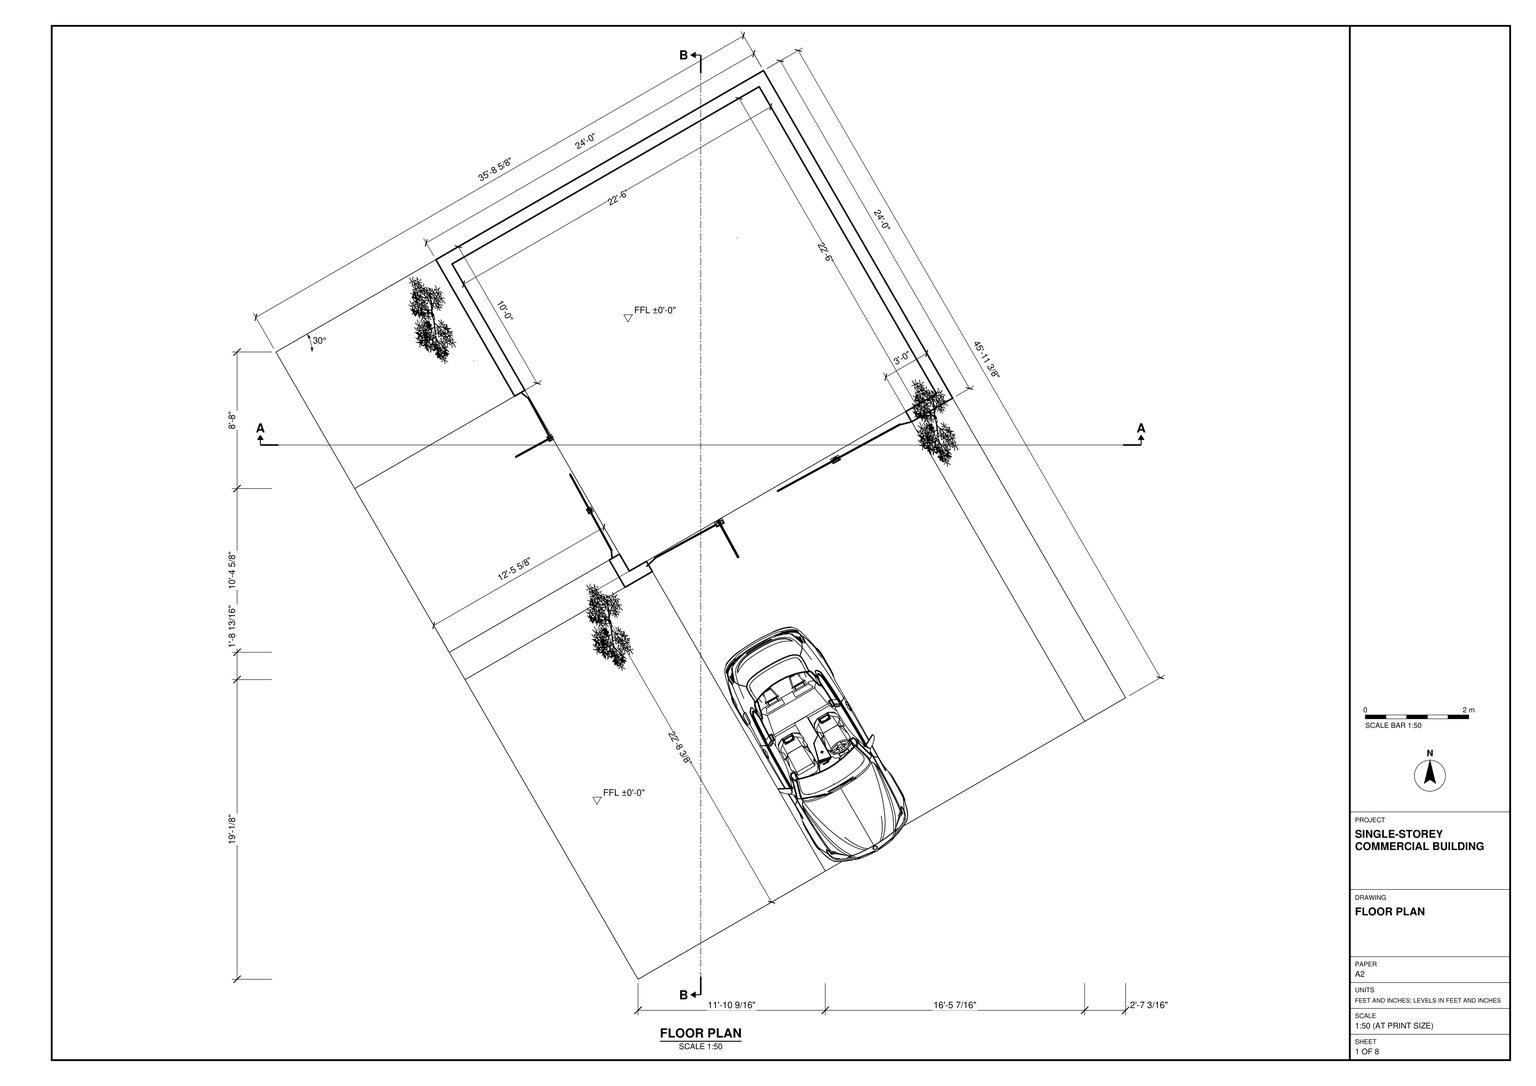
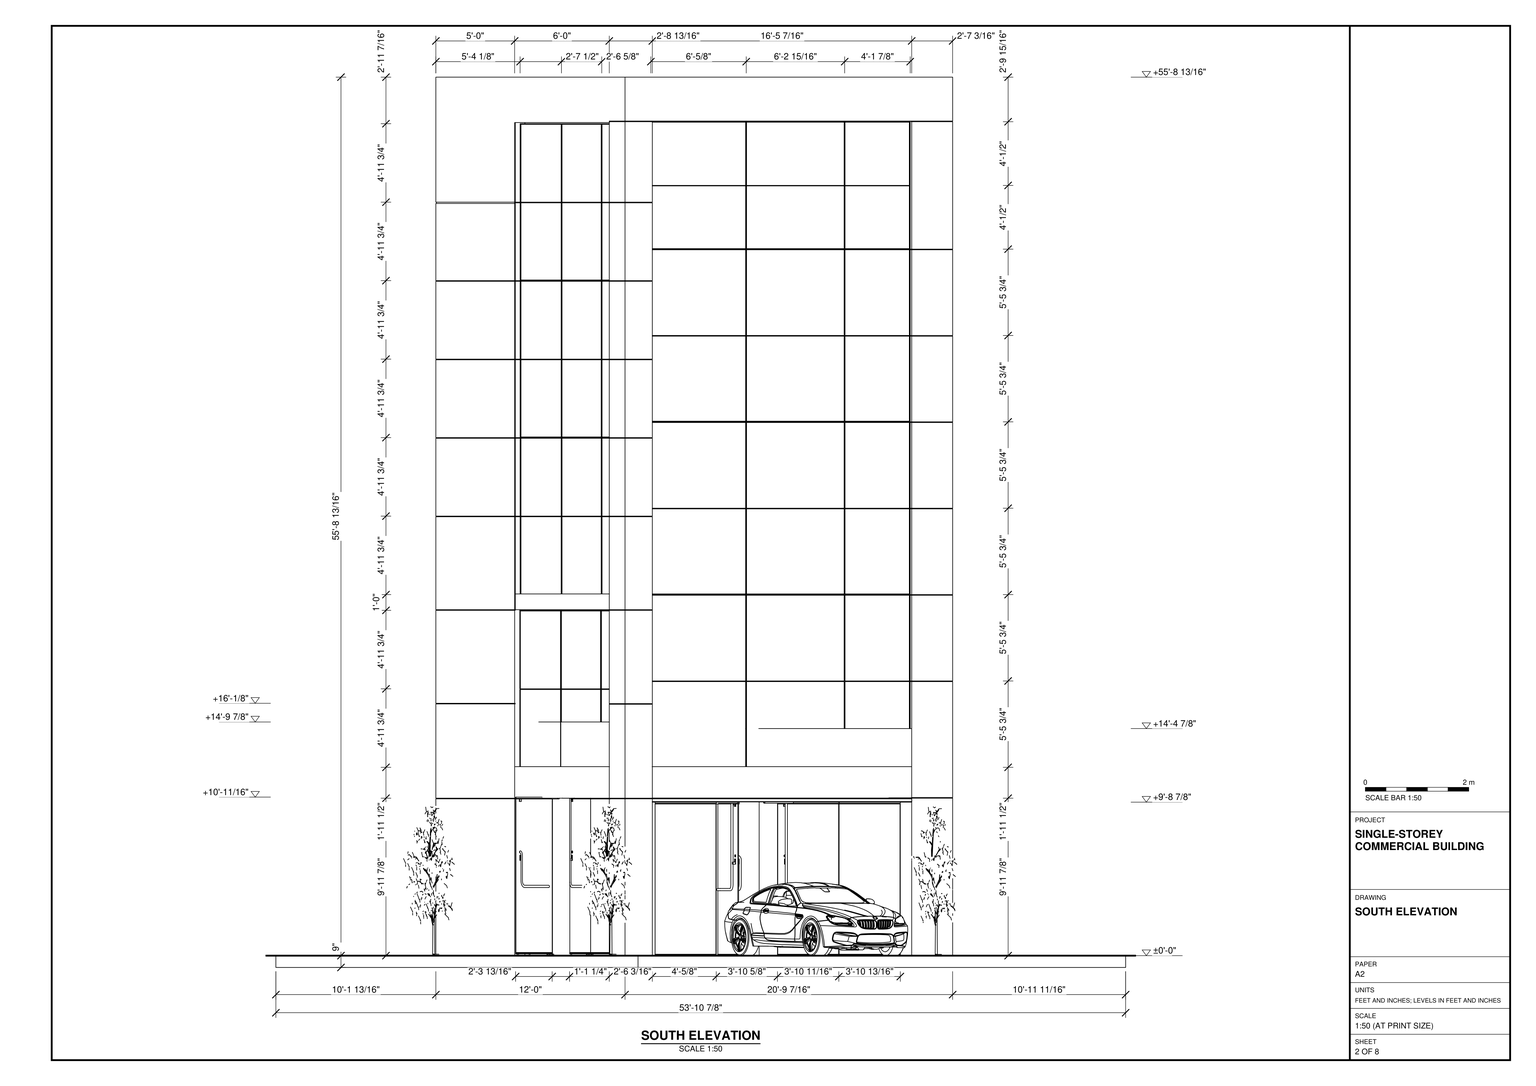
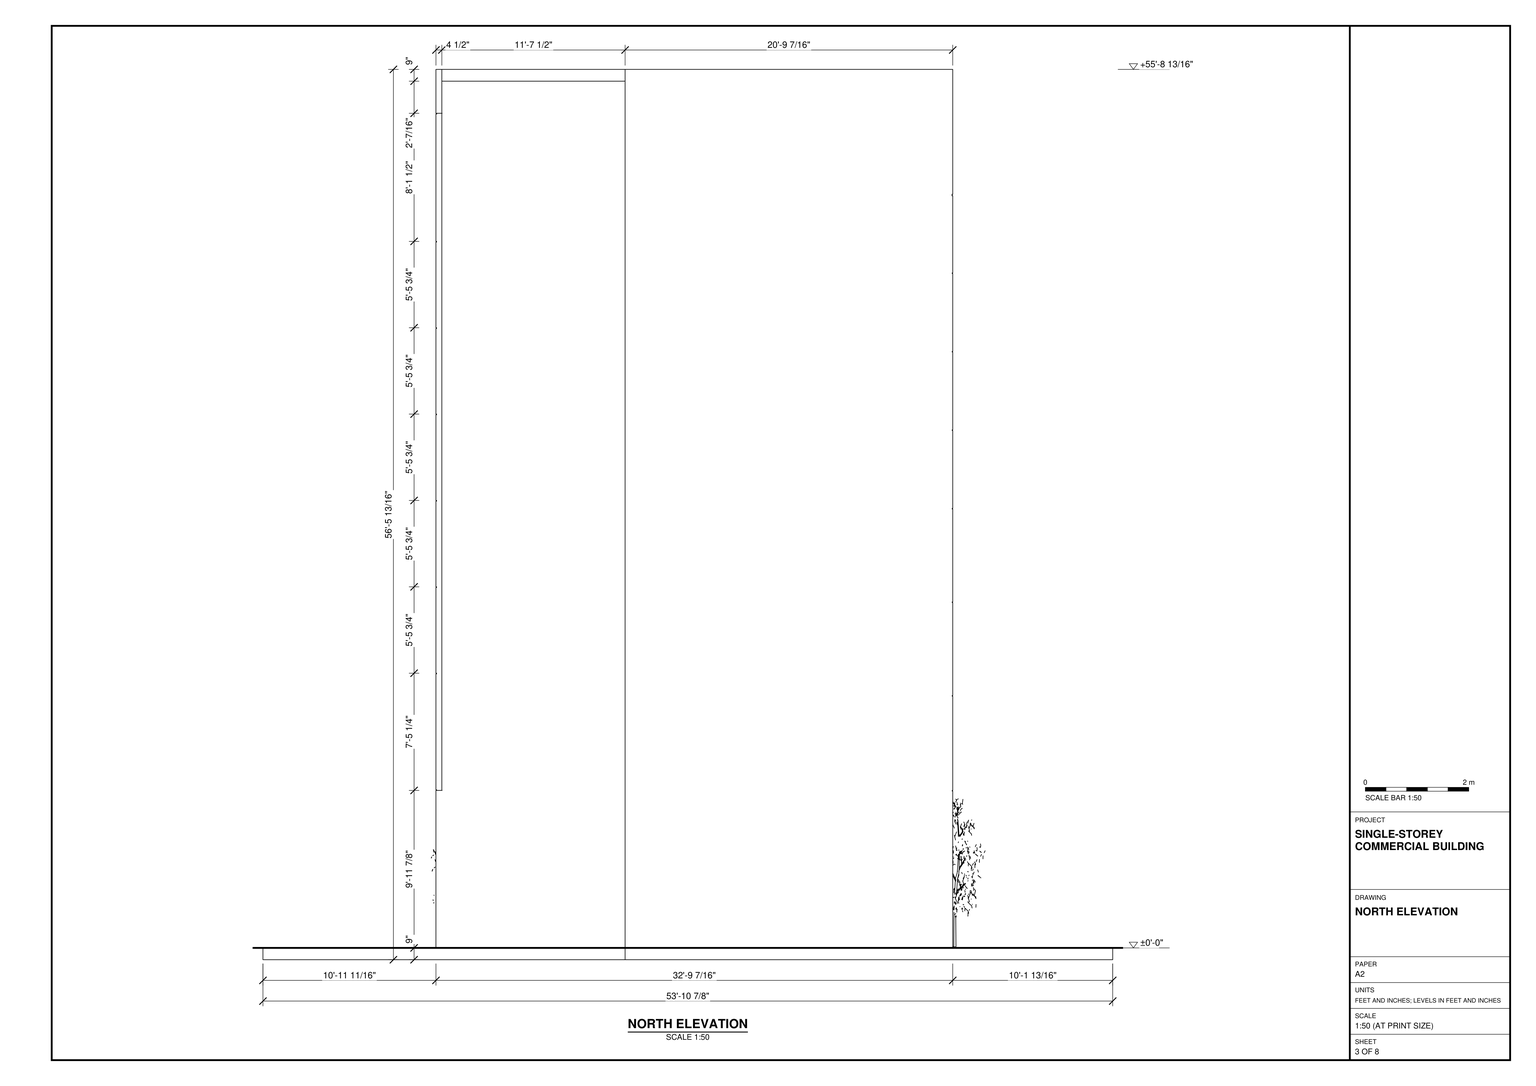
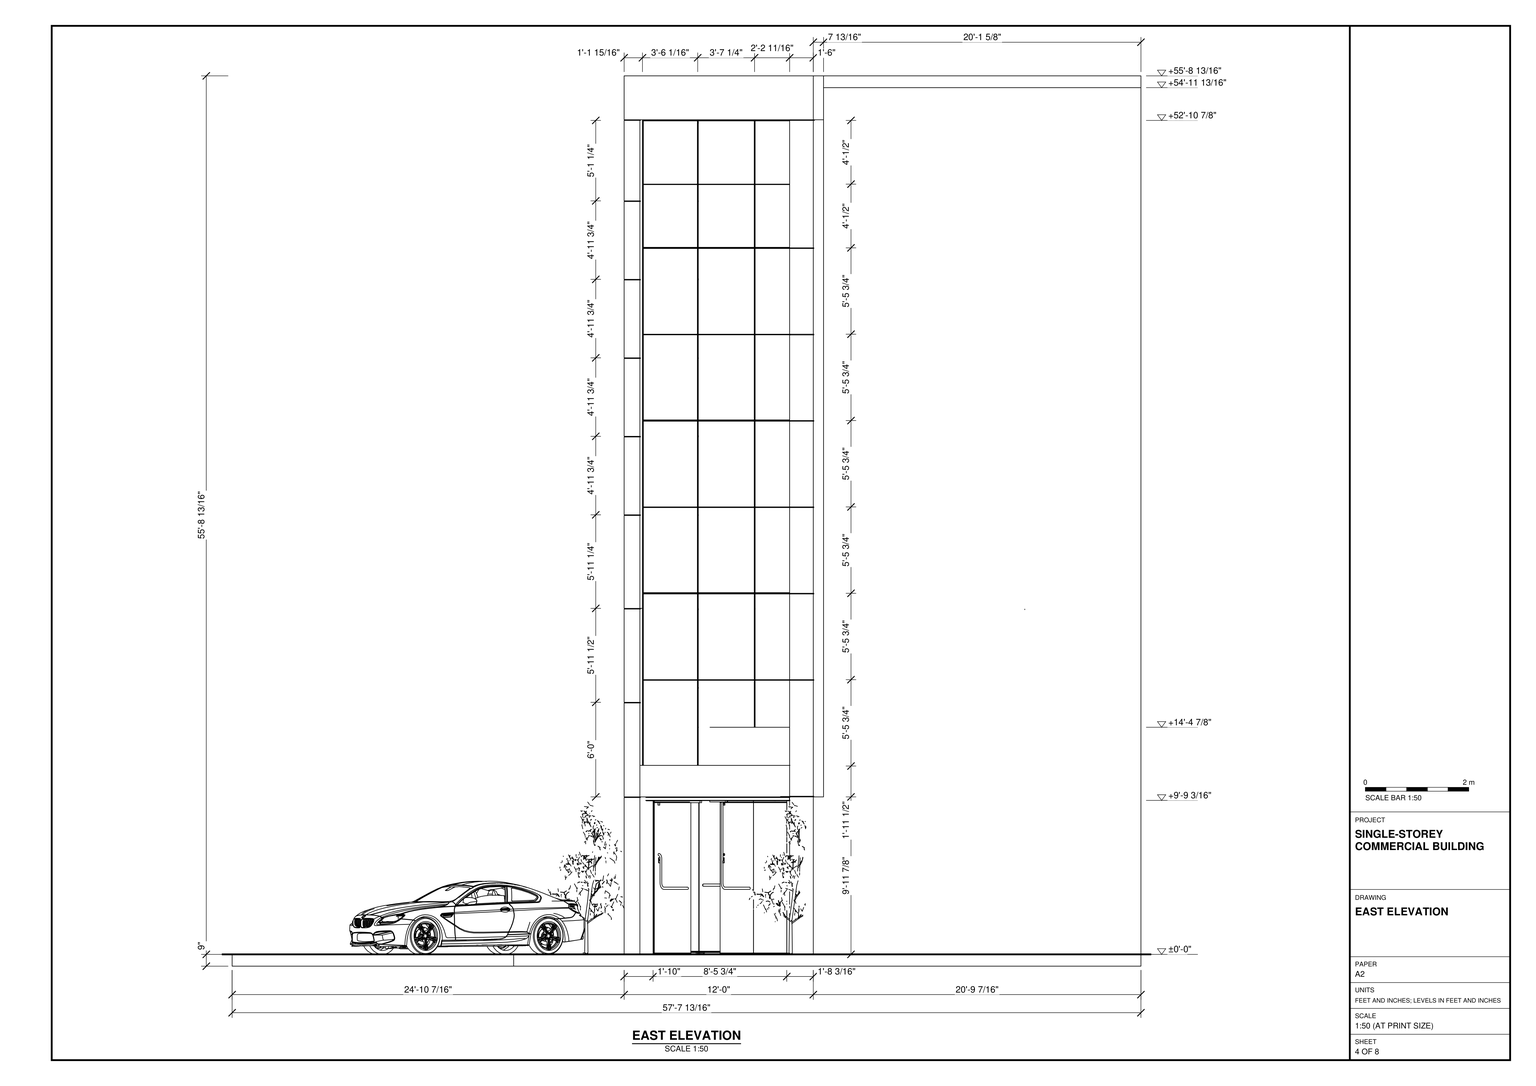
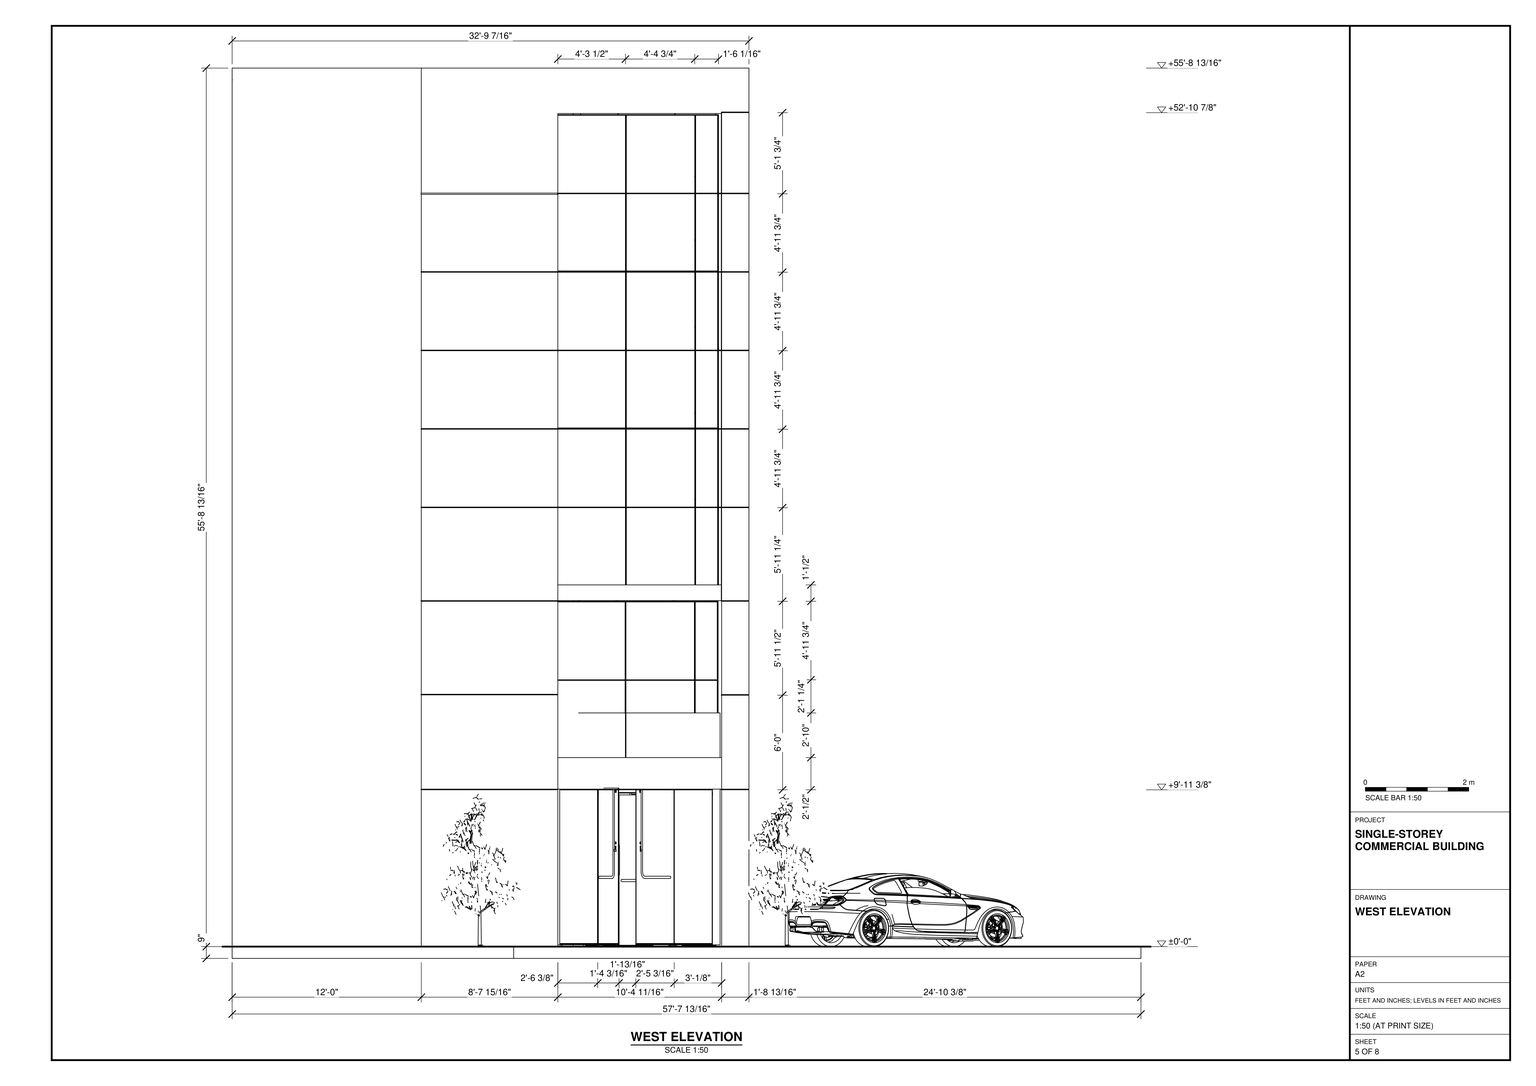
Build the commercial building and its site in SketchUp from task_files/diagram_01.pdf. Work in feet and inches. The overall model extents are 53'-10 7/8" along X, 57'-7 13/16" along Y and 56'-5 13/16" along Z. Set the single finished floor and the top of the surrounding site slab at ±0'-0". The slab extends 9" below that datum; the top of the building is at +55'-8 13/16".

Use the floor plan to orient the square building on the rectangular slab. Keep the building and slab edges parallel to one another and retain their angle to north. Place the building toward the end opposite the parked car, leaving the forecourt and side clearance shown. Model the perimeter walls at their drawn thicknesses, including the short solid wall returns beside the glazed openings.

Use the south elevation to lay out the glazed doors, the framing above them and the solid strips between and around the glazed fields. Match the different bay widths and horizontal divisions on the two adjoining faces. Keep the walls seen from the north largely plain, and follow the level roofline shown. The horizontal divisions in the glazing are not additional storeys.

Decor and loose site items, including the trees and parked car, may be represented by any suitable library components. Keep shell elements such as walls, slabs and roof separate as groups or components, group each furniture or joinery piece separately, and use components for repeated parts. Save one SketchUp model as output_files/commercial_building_with_two_glazed_frontages.skp.

# SketchUp Ruby script. Lengths in inches.
U = 1.inch
M = Sketchup.active_model
def pt(a) = Geom::Point3d.new(a.map { |v| v * U })
def face(e, loops, mat)
  f = e.add_face(loops[0].map { |a| pt(a) })
  loops[1..].each { |l| e.add_face(l.map { |a| pt(a) }).erase! }
  f.material = f.back_material = mat if mat
  f
end
# faces: each face lists its corners as indices into pts; further lists are holes
def faces(e, pts, list, mat = nil) = list.each { |f| face(e, (f[0].is_a?(Array) ? f : [f]).map { |l| l.map { |i| pts[i] } }, mat) }
# xy, xz, yz: faces in a plane at the given z, y or x. An outline is a flat list of corners, or four numbers for a rectangle; further outlines are holes
def ring(l) = l.size == 4 ? [[l[0], l[1]], [l[2], l[1]], [l[2], l[3]], [l[0], l[3]]] : l.each_slice(2).to_a
def flat(e, list, mat, &to3) = list.each { |f| face(e, (f[0].is_a?(Array) ? f : [f]).map { |l| ring(l).map { |u, v| to3.(u, v) } }, mat) }
def xy(e, z, list, mat = nil) = flat(e, list, mat) { |x, y| [x, y, z] }
def xz(e, y, list, mat = nil) = flat(e, list, mat) { |x, z| [x, y, z] }
def yz(e, x, list, mat = nil) = flat(e, list, mat) { |y, z| [x, y, z] }
def lines(e, pts, list) = list.each { |a, b| e.add_line(pt(pts[a]), pt(pts[b])) }
# prism: a flat outline (further loops are holes) pulled along v
def prism(e, loops, v, mat = nil)
  f = face(e, loops, mat); d = Geom::Vector3d.new(v.map { |x| x * U })
  f.pushpull(f.normal.samedirection?(d) ? d.length : -d.length)
end
def box(e, o, s, mat = nil) = prism(e, [[o, [o[0] + s[0], o[1], o[2]], [o[0] + s[0], o[1] + s[1], o[2]], [o[0], o[1] + s[1], o[2]]]], [0, 0, s[2]], mat)
def at(x, y, z, deg = 0) = Geom::Transformation.translation(pt([x, y, z])) * Geom::Transformation.rotation(ORIGIN, Z_AXIS, deg.degrees)
def axes(o, x, y, z) = Geom::Transformation.new([*x, 0, *y, 0, *z, 0, *pt(o).to_a, 1])
def part(name) = M.definitions.add(name)
# library, detail: a bought-in or finely detailed component or shape, given as its bounding box
def library(name, o, s) = part(name).tap { |d| box(d.entities, o, s) }
def detail(e, o, s) = box(e.add_group.entities, o, s)
def put(e, d, t, mat = nil) = e.add_instance(d, t).tap { |i| i.material = mat if mat }
def group(e, t, mat = nil) = e.add_group.tap { |g| g.transformation = t; g.material = mat if mat }.entities
root = M.entities
M.materials.add("Color_006").color = [86, 86, 86]
M.materials.add("Metal_Aluminum_Anodized").color = [202, 209, 219]
M.materials.add("Translucent_Glass_Blue").color = [0, 0, 0]
M.materials["Translucent_Glass_Blue"].alpha = 0.15
M.materials.add("[0060_GrassGreen]").color = [62, 91, 5]
M.materials.add("[0137_Black]").color = [102, 102, 102]
M.materials.add("[Metal Silver]").color = [234, 233, 238]
M.materials.add("[Metal_Corrogated_Shiny]1").color = [0, 0, 0]
M.materials.add("acacia").color = [205, 212, 195]
c1 = library("Flat washer",[0,0,0],[2.37,2.37,0.11])
c2 = library("Square cover plate",[0.66,9.07,0],[4.59,4.59,0.09])
c3 = part("Component\#60")
xy(c3.entities,0,[[1,0,4,4]],"[Metal_Corrogated_Shiny]1")
xy(c3.entities,0.95,[[1.17,0.17,3.83,3.83]],"[Metal_Corrogated_Shiny]1")
xy(c3.entities,3,[[[1,0,4,4],[1.17,0.17,3.83,3.83]]],"[Metal_Corrogated_Shiny]1")
xz(c3.entities,0,[[1,0,4,3]],"[Metal_Corrogated_Shiny]1")
xz(c3.entities,0.17,[[1.17,0.95,3.83,3]],"[Metal_Corrogated_Shiny]1")
xz(c3.entities,3.83,[[1.17,0.95,3.83,3]],"[Metal_Corrogated_Shiny]1")
xz(c3.entities,4,[[1,0,4,3]],"[Metal_Corrogated_Shiny]1")
yz(c3.entities,1,[[0,0,4,3]],"[Metal_Corrogated_Shiny]1")
yz(c3.entities,1.17,[[0.17,0.95,3.83,3]],"[Metal_Corrogated_Shiny]1")
yz(c3.entities,3.83,[[0.17,0.95,3.83,3]],"[Metal_Corrogated_Shiny]1")
yz(c3.entities,4,[[0,0,4,3]],"[Metal_Corrogated_Shiny]1")
c4 = library("Component\#53",[0,0,0],[0.53,0.53,0.125])
c5 = part("Component\#52")
xz(c5.entities,0,[[0.0625,0,5.71,156]],"[Metal_Corrogated_Shiny]1")
xz(c5.entities,0.0625,[[0,0,0.0625,156],[5.71,0,5.77,156]])
xz(c5.entities,0.125,[[0,0,0.0625,156],[5.71,0,5.77,156]])
xz(c5.entities,0.1875,[[0,0,0.0625,156],[5.71,0,5.77,156]])
yz(c5.entities,0,[[0.0625,0,0.125,156]])
yz(c5.entities,0,[[0.1875,0,38.2,156]],"Translucent_Glass_Blue")
yz(c5.entities,0.0625,[[0,0,0.0625,156],[0.125,0,0.1875,156]])
yz(c5.entities,5.71,[[0,0,0.0625,156],[0.125,0,0.1875,156]])
yz(c5.entities,5.77,[[0.0625,0,0.125,156]])
c6 = library("Door frame channel",[0,0,0],[6.25,2.05,156])
c7 = part("Component\#51")
prism(c7.entities,[[[6.09,2,0],[6.09,1.625,0],[6.15,1.625,0],[6.15,0.125,0],[6.09,0.125,0],[6.09,0,0],[0.0625,0,0],[0.0625,0.125,0],[0,0.125,0],[0,1.625,0],[0.0625,1.625,0],[0.0625,2,0],[0.25,2,0],[5.9,2,0]],[[5.96,0.125,0],[5.96,1.875,0],[0.1875,1.875,0],[0.1875,0.125,0]]],[0,0,156],"[Metal_Corrogated_Shiny]1")
c8 = part("Component\#50")
box(c8.entities,[0,0,-3.25],[1.625,0.75,16.75])
c9 = part("Component\#47")
box(c9.entities,[0,0,0],[1.625,1,13.5],"[Metal_Corrogated_Shiny]1")
c10 = library("Component\#49",[0.75,0,0],[0.75,0.5,16.75])
c11 = library("Glass door assembly",[0,0.34,0.3125],[36,6.07,85.9375])
c12 = library("Fixed glazing panel",[0,0,0.8125],[36,0.75,84.4375])
c13 = part("Glass Doors")
p = [[-9.64,246.33,0],[-9.66,246.34,0],[-9.64,246.35,0],[-9.66,246.36,0],[-9.64,246.375,0],[-9.66,246.38,0],
  [-9.64,246.39,0],[-9.66,246.4,0],[-9.64,246.41,0],[-9.66,246.42,0],[-9.64,246.43,0],[-9.66,246.44,0],
  [-9.64,246.45,0]]
lines(c13.entities,p,[[0,1],[1,2],[2,3],[3,4],[4,5],[5,6],[6,7],[7,8],[8,9],[9,10],[10,11],[11,12]])
put(c13.entities,c1,axes([131.42,22.72,-1.61],[0,-1,0],[-1,0,0],[0,0,1]))
put(c13.entities,c2,axes([141.61,24.49,0],[0,-1,0],[-1,0,0],[0,0,1]),"Metal_Aluminum_Anodized")
put(c13.entities,c1,axes([62.98,22.72,-1.61],[0,-1,0],[-1,0,0],[0,0,1]))
put(c13.entities,c2,axes([73.16,24.49,0],[0,-1,0],[-1,0,0],[0,0,1]),"Metal_Aluminum_Anodized")
put(c13.entities,c3,at(59.79,23.6,-3,-90),"Metal_Aluminum_Anodized")
put(c13.entities,c3,at(128.05,23.6,-3,-90),"Metal_Aluminum_Anodized")
put(c13.entities,c1,axes([131.24,22.29,-1.61],[0,-1,0],[-1,0,0],[0,0,1]))
put(c13.entities,c4,at(57.64,21.27,84.4375))
put(c13.entities,c5,axes([18.08,18.65,86.62],[0,1,0],[0,0,1],[1,0,0]),"Metal_Aluminum_Anodized")
put(c13.entities,c6,axes([18.08,18.41,84.5625],[0,1,0],[0,0,1],[1,0,0]),"Metal_Aluminum_Anodized")
put(c13.entities,c7,axes([18.08,18.46,84.62],[0,1,0],[0,0,1],[1,0,0]),"Metal_Aluminum_Anodized")
put(c13.entities,c8,axes([90.95,18.76,83.8125],[0,1,0],[0,0,1],[1,0,0]),"Color_006")
put(c13.entities,c4,at(133.86,21.27,84.4375))
put(c13.entities,c4,at(61.68,21.27,84.4375))
put(c13.entities,c9,axes([118.42,21.99,83.4375],[0,1,0],[0,0,1],[1,0,0]),"Color_006")
put(c13.entities,c9,axes([60.11,21.99,83.4375],[0,1,0],[0,0,1],[1,0,0]),"Color_006")
put(c13.entities,c4,at(129.83,21.27,84.4375))
put(c13.entities,c10,axes([87.7,19.63,83.9375],[0,1,0],[0,0,1],[1,0,0]))
put(c13.entities,c11,at(58.58,23.52,-1.8125,-90))
put(c13.entities,c12,at(23.83,21.16,-0.8125))
put(c13.entities,c12,at(132.2,21.16,-0.8125))
put(c13.entities,c11,axes([132.08,18.32,-1.8125],[-1,0,0],[0,1,0],[0,0,1]))
c14 = part("Glazed frontage")
p = [[33.49,33.64,3.1875],[27.74,31.125,3.1875],[27.74,31.125,87.4375],[33.49,33.64,87.4375],[177.86,33.64,87.4375],[183.74,31.125,87.4375],
  [183.74,31.125,3.1875],[177.86,33.64,3.1875]]
faces(c14.entities,p,[[0,1,2,3],[4,5,6,7]],"[Metal_Corrogated_Shiny]1")
put(c14.entities,c13,at(9.66,12.48,3),"[Metal_Corrogated_Shiny]1")
c15 = library("branch2",[-7.01,-2.24,-3.95],[100.2,82.39,73.03])
c16 = part("mahogany")
p = [[0,6.55,3.76],[16.42,5.72,3.76],[6.78,12.33,0],[7.45,0,0.39]]
faces(c16.entities,p,[[0,1,2],[0,3,1]],"acacia")
c17 = library("trunk_branch",[72.14,-7.82,0],[146.07,127.02,339.64])
c18 = part("acacia")
put(c18.entities,c15,at(159.55,102.76,81.4))
put(c18.entities,c15,at(100.84,178.42,92.02,-177))
put(c18.entities,c15,at(153.14,118.31,162.88,32))
put(c18.entities,c15,axes([182.92,126.14,204.97],[0.60617,0.42445,0],[-0.42445,0.60617,0],[0,0,0.74]))
put(c18.entities,c15,at(140.59,128.21,181.02,-62.186))
put(c18.entities,c15,at(180.63,102.91,109.04,-117))
put(c18.entities,c15,at(127.09,136.92,139.72,153))
put(c18.entities,c15,at(120.34,92.39,197.11,-59.898))
put(c18.entities,c15,at(143.47,146.45,79.95,100))
put(c18.entities,c15,at(120.94,127.28,193.32,-135))
put(c18.entities,c15,axes([114.09,138.74,280.37],[-0.69957,-0.02443,0],[0.02443,-0.69957,0],[0,0,0.7]))
put(c18.entities,c15,axes([136.77,132.09,302.17],[0.23176,0.71329,0],[-0.71329,0.23176,0],[0,0,0.75]))
put(c18.entities,c15,at(112.64,155.99,78.7,-137))
put(c18.entities,c16,at(155.69,128.05,0,45))
put(c18.entities,c15,at(129.34,130.66,223.59,60))
put(c18.entities,c15,at(154.12,121.53,89.82,-117))
put(c18.entities,c15,at(107.69,136.2,139.23,-147))
put(c18.entities,c15,at(105.19,125.71,134.72,-90))
put(c18.entities,c15,axes([187.3,80.72,110.65],[0.71193,-0.51725,0],[0.51725,0.71193,0],[0,0,0.88]))
put(c18.entities,c15,at(128.34,100.5625,202.45,-135))
put(c18.entities,c15,axes([101.26,126.84,280.37],[-0.07317,-0.69617,0],[0.69617,-0.07317,0],[0,0,0.7]))
put(c18.entities,c15,axes([107.73,131.68,316.17],[0.13251,-0.69887,0.23774],[0.73719,0.11263,-0.07979],[0.03865,0.24778,0.70683]))
put(c18.entities,c17,at(0,59.26,2.07))
put(c18.entities,c15,at(124.23,150.7,237.45,90))
put(c18.entities,c15,at(125.7,153.24,222.61,142))
put(c18.entities,c15,axes([117.42,149.09,316],[-0.17154,0.05839,0.72778],[0.10919,-0.73714,0.08488],[0.72191,0.12537,0.1601]))
c19 = library("car",[-8.95,-10.83,0],[83.51,184.88,55.74])
c20 = part("Group\#1")
xz(c20.entities,0,[[[0,0,144,119.5],[0.5,59.75,62.5,119],[0.5,0.5,62.5,59.25],[63,59.75,123.4375,119],[63,0.5,123.4375,59.25],[123.9375,59.75,143.5,119],[123.9375,0.5,143.5,59.25]]])
xz(c20.entities,0.5,[[0.5,0.5,62.5,59.25],[63,0.5,123.4375,59.25],[123.9375,0.5,143.5,59.25],[0.5,59.75,62.5,119],[63,59.75,123.4375,119],
  [123.9375,59.75,143.5,119]],"[0137_Black]")
yz(c20.entities,63,[[0,0.5,0.5,59.25]])
c21 = part("Group\#2")
yz(c21.entities,0,[[0.5,0.5,83.625,65.25],[84.125,0.5,170.1875,65.25],[170.6875,0.5,227.5,65.25],[0.5,65.75,83.625,131],[84.125,65.75,170.1875,131],
  [170.6875,65.75,227.5,131]],"[0137_Black]")
yz(c21.entities,0.5,[[[0,0,228,131.5],[170.6875,0.5,170.6875,65.25,227.5,65.25,227.5,65.75,170.6875,65.75,170.6875,131,227.5,131,227.5,0.5],[84.125,65.75,170.1875,131],[84.125,0.5,170.1875,65.25],[0.5,65.75,83.625,131],[0.5,0.5,83.625,65.25]]])
xy(root,-9,[[275.6875,0,0,477.5,371.2,691.82,646.89,214.3125]])
xy(root,0,[[265.78,298.4,286.57,310.4,282.07,318.2,269.08,310.7,261.58,323.6875,253.78,319.1875],[269.08,310.7,282.07,318.2,479.52,432.2,502.91,445.7,367.91,679.52,134.08,544.52,189.58,448.39,261.58,323.6875]])
xy(root,0,[[275.6875,0,418.26,82.3125,286.57,310.4,265.78,298.4,144,228.09],[418.26,82.3125,615.71,196.3125,484.02,424.4,479.52,432.2,282.07,318.2,286.57,310.4],[144,228.09,265.78,298.4,253.78,319.1875,132,248.875],[132,248.875,253.78,319.1875,261.58,323.6875,189.58,448.39,181.78,443.89,60,373.58],[60,373.58,181.78,443.89,121.78,547.82,0,477.5]],"[Metal Silver]")
xy(root,119.375,[[265.78,298.4,266.65,298.9,266.4,299.33,254.65,319.6875,253.78,319.1875],[266.65,298.9,286.57,310.4,286.32,310.83,266.4,299.33],[181.78,443.89,182.22,444.14,122.22,548.07,121.78,547.82]])
xy(root,119.875,[[265.78,298.4,266.65,298.9,266.4,299.33,254.65,319.6875,253.78,319.1875],[266.65,298.9,286.57,310.4,286.32,310.83,266.4,299.33],[266.4,299.33,286.32,310.83,282.07,318.2,269.08,310.7,261.58,323.6875,254.65,319.6875],[286.57,310.4,286.32,310.83,282.07,318.2,479.52,432.2,483.77,424.83,484.02,424.4],[253.78,319.1875,181.78,443.89,182.22,444.14,189.58,448.39,261.58,323.6875,254.65,319.6875],
  [484.02,424.4,515.2,442.4,514.95,442.83,483.77,424.83],[483.77,424.83,514.95,442.83,510.7,450.2,502.91,445.7,479.52,432.2],[181.78,443.89,121.78,547.82,122.22,548.07,182.22,444.14]])
xy(root,120.375,[[484.02,424.4,483.77,424.83,514.95,442.83,515.2,442.4]])
xy(root,143.375,[[283.89,314.05,283.64,314.48,481.09,428.48,481.34,428.05],[257.43,321.87,185.43,446.58,185.86,446.83,257.86,322.12]])
xy(root,143.875,[[[286.57,310.4,484.02,424.4,479.52,432.2,282.07,318.2,284.07,314.73,356.06,356.29,356.31,355.86,284.32,314.3],[356.74,356.11,356.49,356.54,431.02,399.58,431.27,399.14],[431.71,399.39,431.46,399.83,480.66,428.23,480.91,427.8]],[284.32,314.3,356.31,355.86,356.06,356.29,284.07,314.73],[[253.78,319.1875,261.58,323.6875,189.58,448.39,186.11,446.39,217.11,392.7,216.68,392.45,185.68,446.14,181.78,443.89],[247.15,339.68,216.93,392.02,217.36,392.27,247.58,339.93],[257.18,322.3,247.4,339.24,247.83,339.49,257.61,322.55]],[257.18,322.3,257.61,322.55,247.83,339.49,247.4,339.24],[247.15,339.68,247.58,339.93,217.36,392.27,216.93,392.02],
  [356.74,356.11,431.27,399.14,431.02,399.58,356.49,356.54],[216.68,392.45,217.11,392.7,186.11,446.39,185.68,446.14],[431.71,399.39,480.91,427.8,480.66,428.23,431.46,399.83]])
xy(root,191.375,[[265.78,298.4,266.22,298.65,265.97,299.08,254.22,319.4375,253.78,319.1875],[266.22,298.65,286.57,310.4,286.32,310.83,265.97,299.08]])
xy(root,191.625,[[181.78,443.89,182.22,444.14,122.22,548.07,121.78,547.82]])
xy(root,191.875,[[265.78,298.4,253.78,319.1875,254.22,319.4375,265.97,299.08,266.22,298.65],[266.22,298.65,265.97,299.08,286.32,310.83,286.57,310.4]])
xy(root,192.125,[[181.78,443.89,121.78,547.82,122.22,548.07,182.22,444.14]])
xy(root,202.625,[[257.18,322.3,247.4,339.24,247.83,339.49,257.61,322.55],[247.15,339.68,216.93,392.02,217.36,392.27,247.58,339.93],[216.68,392.45,185.68,446.14,186.11,446.39,217.11,392.7]])
xy(root,203.125,[[257.18,322.3,257.61,322.55,247.83,339.49,247.4,339.24],[247.15,339.68,247.58,339.93,217.36,392.27,216.93,392.02],[216.68,392.45,217.11,392.7,186.11,446.39,185.68,446.14]])
xy(root,208.625,[[284.32,314.3,284.07,314.73,356.06,356.29,356.31,355.86],[356.74,356.11,356.49,356.54,431.02,399.58,431.27,399.14],[431.71,399.39,431.46,399.83,480.66,428.23,480.91,427.8],[484.02,424.4,515.2,442.4,514.95,442.83,483.77,424.83]])
xy(root,209.125,[[284.32,314.3,356.31,355.86,356.06,356.29,284.07,314.73],[356.74,356.11,431.27,399.14,431.02,399.58,356.49,356.54],[431.71,399.39,480.47,427.55,480.22,427.98,431.46,399.83],[484.02,424.4,483.77,424.83,514.95,442.83,515.2,442.4],[480.47,427.55,480.91,427.8,480.66,428.23,480.22,427.98]])
xy(root,262.375,[[257.18,322.3,247.4,339.24,247.83,339.49,257.61,322.55],[247.15,339.68,216.93,392.02,217.36,392.27,247.58,339.93],[216.68,392.45,185.68,446.14,186.11,446.39,217.11,392.7]])
xy(root,262.875,[[265.78,298.4,266.22,298.65,265.97,299.08,254.22,319.4375,253.78,319.1875],[266.22,298.65,286.57,310.4,286.32,310.83,265.97,299.08],[257.43,321.87,257.86,322.12,185.86,446.83,185.43,446.58],[181.78,443.89,182.22,444.14,122.22,548.07,121.78,547.82]])
xy(root,263.375,[[265.78,298.4,253.78,319.1875,254.22,319.4375,265.97,299.08,266.22,298.65],[266.22,298.65,265.97,299.08,286.32,310.83,286.57,310.4],[265.97,299.08,254.22,319.4375,254.26,319.46,261.58,323.6875,269.08,310.7,282.07,318.2,284.07,314.73,284.32,314.3,286.32,310.83],[254.26,319.46,182.26,444.17,189.58,448.39,261.58,323.6875],[181.78,443.89,121.78,547.82,122.22,548.07,182.22,444.14]])
xy(root,274.375,[[284.32,314.3,284.07,314.73,356.06,356.29,356.31,355.86],[356.74,356.11,356.49,356.54,431.02,399.58,431.27,399.14],[431.71,399.39,431.46,399.83,480.66,428.23,480.91,427.8],[484.02,424.4,515.2,442.4,514.95,442.83,483.77,424.83]])
xy(root,274.875,[[283.89,314.05,481.34,428.05,481.09,428.48,283.64,314.48],[484.02,424.4,483.77,424.83,514.95,442.83,515.2,442.4]])
xy(root,275.375,[[254.26,319.46,261.58,323.6875,189.58,448.39,182.26,444.17]])
xy(root,334.125,[[265.78,298.4,266.22,298.65,265.97,299.08,254.22,319.4375,253.78,319.1875],[266.22,298.65,286.57,310.4,286.32,310.83,265.97,299.08],[181.78,443.89,182.22,444.14,122.22,548.07,121.78,547.82]])
xy(root,334.625,[[265.78,298.4,253.78,319.1875,254.22,319.4375,265.97,299.08,266.22,298.65],[266.22,298.65,265.97,299.08,286.32,310.83,286.57,310.4],[181.78,443.89,121.78,547.82,122.22,548.07,182.22,444.14]])
xy(root,340.14,[[484.02,424.4,515.2,442.4,514.95,442.83,483.77,424.83]])
xy(root,340.625,[[484.02,424.4,483.77,424.83,514.95,442.83,515.2,442.4]])
xy(root,393.875,[[265.78,298.4,266.22,298.65,265.97,299.08,254.22,319.4375,253.78,319.1875],[266.22,298.65,286.57,310.4,286.32,310.83,265.97,299.08],[181.78,443.89,182.22,444.14,122.22,548.07,121.78,547.82]])
xy(root,394.375,[[265.78,298.4,253.78,319.1875,254.22,319.4375,265.97,299.08,266.22,298.65],[266.22,298.65,265.97,299.08,286.32,310.83,286.57,310.4],[181.78,443.89,121.78,547.82,122.22,548.07,182.22,444.14]])
xy(root,405.875,[[484.02,424.4,515.2,442.4,514.95,442.83,483.77,424.83]])
xy(root,406.375,[[484.02,424.4,483.77,424.83,514.95,442.83,515.2,442.4]])
xy(root,453.625,[[265.78,298.4,266.26,298.68,266.01,299.11,254.26,319.46,253.78,319.1875],[266.26,298.68,286.57,310.4,286.32,310.83,266.01,299.11],[181.78,443.89,182.22,444.14,122.22,548.07,121.78,547.82]])
xy(root,454.125,[[265.78,298.4,253.78,319.1875,254.26,319.46,266.01,299.11,266.26,298.68],[266.26,298.68,266.01,299.11,286.32,310.83,286.57,310.4],[181.78,443.89,121.78,547.82,122.22,548.07,182.22,444.14]])
xy(root,471.55,[[484.02,424.4,515.2,442.4,514.95,442.83,483.77,424.83]])
xy(root,472.125,[[484.02,424.4,483.77,424.83,514.95,442.83,515.2,442.4]])
xy(root,513.375,[[265.78,298.4,266.26,298.68,266.01,299.11,254.26,319.46,253.78,319.1875],[266.26,298.68,286.57,310.4,286.32,310.83,266.01,299.11],[181.78,443.89,182.22,444.14,122.22,548.07,121.78,547.82]])
xy(root,513.875,[[265.78,298.4,253.78,319.1875,254.26,319.46,266.01,299.11,266.26,298.68],[266.26,298.68,266.01,299.11,286.32,310.83,286.57,310.4],[181.78,443.89,121.78,547.82,122.22,548.07,182.22,444.14]])
xy(root,537.375,[[484.02,424.4,515.2,442.4,514.95,442.83,483.77,424.83]])
xy(root,537.875,[[484.02,424.4,483.77,424.83,514.95,442.83,515.2,442.4]])
xy(root,572.65,[[181.78,443.89,182.26,444.17,122.26,548.09,121.78,547.82]])
xy(root,573.125,[[265.78,298.4,265.95,298.5,265.7,298.93,253.95,319.28,253.78,319.1875],[265.95,298.5,286.57,310.4,286.32,310.83,265.7,298.93]])
xy(root,573.625,[[265.78,298.4,253.78,319.1875,253.95,319.28,265.7,298.93,265.95,298.5],[265.95,298.5,265.7,298.93,286.32,310.83,286.57,310.4],[181.78,443.89,121.78,547.82,122.26,548.09,182.26,444.17]])
xy(root,634.25,[[253.78,319.1875,181.78,443.89,182.26,444.17,254.26,319.46],[254.26,319.46,182.26,444.17,189.58,448.39,261.58,323.6875]])
xy(root,634.875,[[265.78,298.4,266.22,298.65,265.97,299.08,254.22,319.4375,253.78,319.1875],[266.22,298.65,286.57,310.4,286.32,310.83,265.97,299.08],[484.02,424.4,515.2,442.4,514.7,443.27,483.52,425.27]])
xy(root,635.375,[[265.78,298.4,266.22,298.65,265.97,299.08,254.22,319.4375,253.78,319.1875],[266.22,298.65,266.26,298.68,266.01,299.11,265.97,299.08],[266.26,298.68,286.57,310.4,286.32,310.83,266.01,299.11],[265.97,299.08,266.01,299.11,254.26,319.46,254.22,319.4375],[266.01,299.11,286.32,310.83,282.07,318.2,269.08,310.7,261.58,323.6875,254.26,319.46],
  [286.57,310.4,286.32,310.83,282.07,318.2,479.52,432.2,483.52,425.27,484.02,424.4],[484.02,424.4,483.52,425.27,514.7,443.27,515.2,442.4]])
xy(root,659.8125,[[269.08,310.7,134.08,544.52,367.91,679.52,502.91,445.7],[502.91,445.7,367.91,679.52,375.7,684.02,510.7,450.2]])
xy(root,668.8125,[[265.78,298.4,515.2,442.4,510.7,450.2,261.28,306.2],[261.28,306.2,510.7,450.2,371.2,691.82,121.78,547.82]])
# 34 loose lines left out
p = [[0,477.5,-9],[275.6875,0,-9],[275.6875,0,0],[144,228.09,0],[132,248.875,0],[60,373.58,0],
  [0,477.5,0],[646.89,214.3125,-9],[646.89,214.3125,-0.14],[615.71,196.3125,0],[418.26,82.3125,0],[371.2,691.82,-9],
  [371.2,691.82,659.8125],[375.7,684.02,659.8125],[510.7,450.2,659.8125],[510.7,450.2,635.375],[510.7,450.2,119.875],[514.95,442.83,119.875],
  [515.2,442.4,119.875],[515.2,442.4,-0.14],[121.78,547.82,0],[121.78,547.82,119.375],[122.22,548.07,119.375],[122.22,548.07,119.875],
  [121.78,547.82,119.875],[121.78,547.82,191.625],[122.22,548.07,191.625],[122.22,548.07,192.125],[121.78,547.82,192.125],[121.78,547.82,262.875],
  [122.22,548.07,262.875],[122.22,548.07,263.375],[121.78,547.82,263.375],[121.78,547.82,334.125],[122.22,548.07,334.125],[122.22,548.07,334.625],
  [121.78,547.82,334.625],[121.78,547.82,393.875],[122.22,548.07,393.875],[122.22,548.07,394.375],[121.78,547.82,394.375],[121.78,547.82,453.625],
  [122.22,548.07,453.625],[122.22,548.07,454.125],[121.78,547.82,454.125],[121.78,547.82,513.375],[122.22,548.07,513.375],[122.22,548.07,513.875],
  [121.78,547.82,513.875],[121.78,547.82,572.65],[122.26,548.09,572.65],[122.26,548.09,573.625],[121.78,547.82,573.625],[121.78,547.82,668.8125],
  [371.2,691.82,668.8125],[484.02,424.4,0],[484.02,424.4,119.875],[253.78,319.1875,119.375],[253.78,319.1875,0],[265.78,298.4,0],
  [265.78,298.4,119.375],[286.57,310.4,0],[286.57,310.4,119.375],[266.65,298.9,119.375],[282.07,318.2,0],[282.07,318.2,119.875],
  [286.32,310.83,119.875],[286.32,310.83,119.375],[134.08,544.52,0],[134.08,544.52,659.8125],[269.08,310.7,659.8125],[269.08,310.7,635.375],
  [269.08,310.7,263.375],[269.08,310.7,119.875],[261.58,323.6875,119.875],[189.58,448.39,119.875],[189.58,448.39,0],[261.58,323.6875,275.375],
  [261.58,323.6875,634.25],[189.58,448.39,634.25],[189.58,448.39,275.375],[261.58,323.6875,143.875],[261.58,323.6875,263.375],[189.58,448.39,263.375],
  [189.58,448.39,143.875],[269.08,310.7,0],[261.58,323.6875,0],[254.65,319.6875,119.375],[254.65,319.6875,119.875],[479.52,432.2,0],
  [483.77,424.83,119.875],[479.52,432.2,119.875],[502.91,445.7,0],[502.91,445.7,119.875],[181.78,443.89,0],[181.78,443.89,119.375],
  [182.22,444.14,119.875],[182.22,444.14,119.375],[367.91,679.52,0],[502.91,445.7,635.375],[502.91,445.7,659.8125],[367.91,679.52,659.8125],
  [266.4,299.33,119.375],[266.4,299.33,119.875],[265.78,298.4,119.875],[265.78,298.4,191.375],[253.78,319.1875,191.375],[253.78,319.1875,143.875],
  [253.78,319.1875,119.875],[286.57,310.4,143.875],[286.57,310.4,191.375],[266.22,298.65,191.375],[266.65,298.9,119.875],[286.57,310.4,119.875],
  [484.02,424.4,120.375],[484.02,424.4,143.875],[479.52,432.2,635.375],[282.07,318.2,263.375],[282.07,318.2,143.875],[479.52,432.2,143.875],
  [181.78,443.89,119.875],[181.78,443.89,143.875],[483.77,424.83,120.375],[514.95,442.83,120.375],[514.7,443.27,635.375],[514.7,443.27,634.875],
  [515.2,442.4,634.875],[515.2,442.4,537.875],[514.95,442.83,537.875],[514.95,442.83,537.375],[515.2,442.4,537.375],[515.2,442.4,472.125],
  [514.95,442.83,472.125],[514.95,442.83,471.55],[515.2,442.4,471.55],[515.2,442.4,406.375],[514.95,442.83,406.375],[514.95,442.83,405.875],
  [515.2,442.4,405.875],[515.2,442.4,340.625],[514.95,442.83,340.625],[514.95,442.83,340.14],[515.2,442.4,340.14],[515.2,442.4,274.875],
  [514.95,442.83,274.875],[514.95,442.83,274.375],[515.2,442.4,274.375],[515.2,442.4,209.125],[514.95,442.83,209.125],[514.95,442.83,208.625],
  [515.2,442.4,208.625],[515.2,442.4,120.375],[181.78,443.89,191.625],[484.02,424.4,208.625],[283.64,314.48,274.875],[283.64,314.48,143.375],
  [283.89,314.05,143.375],[283.89,314.05,274.875],[481.09,428.48,274.875],[481.09,428.48,143.375],[431.46,399.83,143.875],[480.66,428.23,143.875],
  [480.66,428.23,208.625],[480.66,428.23,209.125],[480.66,428.23,274.375],[431.46,399.83,274.375],[431.46,399.83,209.125],[480.22,427.98,209.125],
  [431.46,399.83,208.625],[356.49,356.54,274.375],[356.49,356.54,209.125],[431.02,399.58,209.125],[431.02,399.58,274.375],[431.02,399.58,208.625],
  [356.49,356.54,208.625],[356.49,356.54,143.875],[431.02,399.58,143.875],[356.06,356.29,274.375],[284.07,314.73,274.375],[284.07,314.73,263.375],
  [284.07,314.73,209.125],[356.06,356.29,209.125],[284.07,314.73,208.625],[284.07,314.73,191.375],[284.07,314.73,190.875],[284.07,314.73,143.875],
  [356.06,356.29,143.875],[356.06,356.29,208.625],[257.86,322.12,143.375],[257.86,322.12,190.875],[257.43,321.87,190.875],[257.43,321.87,143.375],
  [185.86,446.83,262.875],[257.86,322.12,262.875],[185.86,446.83,143.375],[186.11,446.39,203.125],[217.11,392.7,203.125],[217.11,392.7,262.375],
  [186.11,446.39,262.375],[217.11,392.7,202.625],[186.11,446.39,202.625],[186.11,446.39,191.625],[186.11,446.39,191.125],[186.11,446.39,143.875],
  [217.11,392.7,143.875],[217.36,392.27,262.375],[217.36,392.27,203.125],[247.58,339.93,203.125],[247.58,339.93,262.375],[217.36,392.27,143.875],
  [247.58,339.93,143.875],[247.58,339.93,202.625],[217.36,392.27,202.625],[247.83,339.49,262.375],[247.83,339.49,203.125],[257.61,322.55,203.125],
  [257.61,322.55,262.375],[247.83,339.49,143.875],[257.61,322.55,143.875],[257.61,322.55,190.875],[257.61,322.55,191.375],[257.61,322.55,202.625],
  [247.83,339.49,202.625],[481.34,428.05,274.875],[481.34,428.05,143.375],[185.43,446.58,143.375],[185.43,446.58,262.875],[284.32,314.3,143.875],
  [284.32,314.3,190.875],[284.32,314.3,191.375],[284.32,314.3,208.625],[284.32,314.3,209.125],[284.32,314.3,263.375],[286.32,310.83,263.375],
  [286.32,310.83,262.875],[286.57,310.4,262.875],[286.57,310.4,191.875],[286.32,310.83,191.875],[286.32,310.83,191.375],[254.22,319.4375,191.375],
  [254.22,319.4375,191.875],[253.78,319.1875,191.875],[253.78,319.1875,262.875],[254.22,319.4375,262.875],[254.22,319.4375,263.375],[254.26,319.46,263.375],
  [257.18,322.3,143.875],[257.18,322.3,190.875],[247.4,339.24,202.625],[247.4,339.24,143.875],[247.15,339.68,143.875],[247.15,339.68,202.625],
  [356.31,355.86,143.875],[356.31,355.86,208.625],[356.74,356.11,208.625],[356.74,356.11,143.875],[216.68,392.45,143.875],[216.68,392.45,202.625],
  [431.27,399.14,143.875],[431.27,399.14,208.625],[431.71,399.39,208.625],[431.71,399.39,143.875],[483.77,424.83,208.625],[483.77,424.83,209.125],
  [484.02,424.4,209.125],[484.02,424.4,274.375],[483.77,424.83,274.375],[483.77,424.83,274.875],[484.02,424.4,274.875],[484.02,424.4,340.125],
  [484.02,424.4,340.14],[483.77,424.83,340.14],[483.77,424.83,340.625],[484.02,424.4,340.625],[484.02,424.4,405.875],[483.77,424.83,405.875],
  [483.77,424.83,406.375],[484.02,424.4,406.375],[484.02,424.4,471.55],[483.77,424.83,471.55],[483.77,424.83,471.625],[483.77,424.83,472.125],
  [484.02,424.4,472.125],[484.02,424.4,537.375],[483.77,424.83,537.375],[483.77,424.83,537.875],[484.02,424.4,537.875],[484.02,424.4,634.875],
  [483.52,425.27,634.875],[483.52,425.27,635.375],[480.91,427.8,143.875],[480.91,427.8,208.625],[185.68,446.14,143.875],[185.68,446.14,191.125],
  [185.68,446.14,191.625],[185.68,446.14,202.625],[182.26,444.17,263.375],[182.22,444.14,263.375],[182.22,444.14,262.875],[181.78,443.89,262.875],
  [181.78,443.89,192.125],[182.22,444.14,192.125],[182.22,444.14,191.625],[185.68,446.14,203.125],[185.68,446.14,262.375],[257.43,321.87,262.875],
  [257.18,322.3,191.375],[265.97,299.08,191.375],[265.97,299.08,191.875],[257.18,322.3,202.625],[265.78,298.4,191.875],[265.78,298.4,262.875],
  [266.22,298.65,191.875],[266.22,298.65,262.875],[257.18,322.3,203.125],[257.18,322.3,262.375],[247.4,339.24,262.375],[247.4,339.24,203.125],
  [247.15,339.68,203.125],[247.15,339.68,262.375],[216.93,392.02,262.375],[216.93,392.02,203.125],[216.68,392.45,203.125],[216.68,392.45,262.375],
  [480.91,427.8,209.125],[356.31,355.86,209.125],[356.31,355.86,274.375],[356.74,356.11,274.375],[356.74,356.11,209.125],[431.27,399.14,209.125],
  [431.27,399.14,274.375],[431.71,399.39,274.375],[431.71,399.39,209.125],[480.91,427.8,274.375],[265.97,299.08,262.875],[265.97,299.08,263.375],
  [286.57,310.4,263.375],[253.78,319.1875,263.375],[265.78,298.4,263.375],[265.78,298.4,334.125],[253.78,319.1875,334.125],[286.57,310.4,334.125],
  [266.22,298.65,334.125],[266.22,298.65,263.375],[284.32,314.3,274.375],[282.07,318.2,635.375],[286.32,310.83,635.375],[286.32,310.83,634.875],
  [286.57,310.4,634.875],[286.57,310.4,573.625],[286.32,310.83,573.625],[286.32,310.83,573.125],[286.57,310.4,573.125],[286.57,310.4,513.875],
  [286.32,310.83,513.875],[286.32,310.83,513.375],[286.57,310.4,513.375],[286.57,310.4,454.125],[286.32,310.83,454.125],[286.32,310.83,453.625],
  [286.57,310.4,453.625],[286.57,310.4,394.375],[286.32,310.83,394.375],[286.32,310.83,393.875],[286.57,310.4,393.875],[286.57,310.4,334.625],
  [286.32,310.83,334.625],[286.32,310.83,334.125],[253.78,319.1875,334.625],[253.78,319.1875,393.875],[254.22,319.4375,393.875],[254.26,319.46,393.875],
  [254.26,319.46,275.375],[254.22,319.4375,334.125],[254.22,319.4375,334.625],[182.26,444.17,275.375],[181.78,443.89,263.375],[181.78,443.89,334.125],
  [182.26,444.17,334.125],[182.22,444.14,334.125],[254.26,319.46,573.625],[254.26,319.46,634.25],[257.92,321.57,393.875],[257.92,321.57,394.375],
  [254.26,319.46,394.375],[254.26,319.46,453.625],[254.26,319.46,454.125],[254.26,319.46,513.375],[254.26,319.46,513.875],[254.26,319.46,573.125],
  [182.26,444.17,634.25],[182.26,444.17,573.625],[182.26,444.17,572.65],[182.26,444.17,513.875],[182.26,444.17,513.375],[182.26,444.17,454.125],
  [182.26,444.17,453.625],[182.26,444.17,394.375],[182.26,444.17,393.875],[182.26,444.17,334.625],[265.97,299.08,334.125],[265.97,299.08,334.625],
  [182.22,444.14,334.625],[265.78,298.4,334.625],[265.78,298.4,393.875],[266.22,298.65,393.875],[266.22,298.65,334.625],[181.78,443.89,334.625],
  [181.78,443.89,393.875],[182.22,444.14,393.875],[265.97,299.08,393.875],[265.97,299.08,394.375],[254.22,319.4375,394.375],[182.22,444.14,394.375],
  [265.78,298.4,394.375],[265.78,298.4,453.625],[253.78,319.1875,453.625],[253.78,319.1875,394.375],[266.26,298.68,453.625],[266.22,298.65,394.375],
  [181.78,443.89,394.375],[181.78,443.89,453.625],[182.22,444.14,453.625],[266.01,299.11,453.625],[266.01,299.11,454.125],[182.22,444.14,454.125],
  [265.78,298.4,454.125],[265.78,298.4,513.375],[253.78,319.1875,513.375],[253.78,319.1875,454.125],[266.26,298.68,513.375],[266.26,298.68,454.125],
  [181.78,443.89,454.125],[181.78,443.89,513.375],[182.22,444.14,513.375],[266.01,299.11,513.375],[266.01,299.11,513.875],[182.22,444.14,513.875],
  [265.78,298.4,513.875],[265.78,298.4,573.125],[253.78,319.1875,573.125],[253.78,319.1875,513.875],[266.26,298.68,513.875],[265.95,298.5,573.125],
  [253.95,319.28,573.125],[181.78,443.89,513.875],[181.78,443.89,572.65],[265.7,298.93,573.125],[265.7,298.93,573.625],[253.95,319.28,573.625],
  [181.78,443.89,573.625],[181.78,443.89,634.25],[253.78,319.1875,634.25],[253.78,319.1875,634.875],[253.78,319.1875,635.375],[265.78,298.4,635.375],
  [265.78,298.4,668.8125],[261.28,306.2,668.8125],[265.78,298.4,573.625],[265.78,298.4,634.875],[253.78,319.1875,573.625],[266.22,298.65,634.875],
  [265.95,298.5,573.625],[254.26,319.46,635.375],[254.22,319.4375,635.375],[254.22,319.4375,634.875],[261.58,323.6875,635.375],[265.97,299.08,634.875],
  [265.97,299.08,635.375],[266.01,299.11,635.375],[266.22,298.65,635.375],[266.26,298.68,635.375],[286.57,310.4,635.375],[484.02,424.4,635.375],
  [515.2,442.4,635.375],[515.2,442.4,668.8125],[510.7,450.2,668.8125]]
faces(root,p,[[0,1,2,3,4,5,6],[7,8,9,10,2,1],[11,12,13,14,15,16,17,18,19,8,7],[12,11,0,6,20,21,22,23,24,25,26,27,28,29,30,31,32,33,34,35,36,37,38,39,40,41,42,43,44,45,46,47,48,49,50,51,52,53,54],[56,55,19,18],[61,64,65,66,67,62],[[68,69,70,71,72,73,74,75,76],[77,78,79,80],[81,82,83,84]],[85,86,74,73],
  [64,85,73,65],[86,58,57,87,88,74],[89,55,56,90,91],[92,89,91,93],[76,75,96,97,95,94],[98,92,93,99,100,101],[68,98,101,69],[88,87,102,103],
  [103,102,67,66],[23,22,97,96],[113,56,114,115,109],[116,99,93,91,65,73,72,117,118,119],[120,108,107,121],[114,56,90,122],[17,123,122,90],[17,16,15,124,125,126,127,128,129,130,131,132,133,134,135,136,137,138,139,140,141,142,143,144,145,146,147,148,149,150,151,123],
  [93,16,15,99],[154,155,156,157],[[158,159,155,154],[160,161,162,163,164,165,166,167,163,162,168],[169,170,171,172],[173,174,175,176],[177,178,179,180,181],[182,183,184,185,186,187]],[188,189,190,191],[[192,193,189,188,194],[195,196,197,198],[199,200,201,202,203,204],[205,206,207,208],[209,210,211,212],[213,214,215,216],[217,218,219,220,221,222]],[159,158,223,224],[192,194,225,226],[227,228,229,230,182,183,184,185,118,117,179,180,231,232,233,234,235,236,237,238,110,109],
  [185,184,228,227],[81,107,106,239,240,241,242,243,244,245,82],[219,218,246,247],[217,222,248,249],[211,210,250,251],[187,186,252,253],[175,174,254,255],[199,204,256,257],
  [173,176,258,259],[160,168,260,261],[119,115,153,262,263,264,265,266,267,268,269,270,271,272,273,274,275,276,277,278,279,280,281,282,283,284,285,286,287,288,289,116],[162,161,290,291],[[292,293,294,295,200,201,202,203,84,83,296,297,298,299,300,301,302,152,121],[198,195,303,304]],[203,202,293,292],[184,183,229,228],[189,193,305,190],
  [220,219,247,306],[202,201,294,293],[239,307,308,240],[237,308,307,238],[236,110,238,237],[183,182,230,229],[106,241,240,239],[221,220,306,309],
  [300,152,302,301],[302,301,27,26],[201,200,295,294],[216,215,314,315],[214,213,316,317],[208,207,318,319],[206,205,320,321],[197,196,322,323],
  [195,198,304,303],[149,148,263,262],[163,162,291,324],[179,232,231,180],[177,181,325,326],[170,169,327,328],[172,171,329,330],[166,165,331,332],
  [164,163,324,333],[244,243,334,335],[233,335,334,234],[336,235,234,233],[242,337,244,243],[31,30,298,297],[233,232,344,178,179,117,345,346,347,348,349,350,351,352,353,354,355,356,357,358,359,360,361,362,363,364,365,366,367,341,336],[72,71,345,117],
  [344,232,179,178],[368,369,370,371,372,245,244,337,340,373,374],[296,245,372,375],[375,378,379,377,376,297,296],[267,266,145,144],[380,381,78,77,372,371,382,383,384,385,386,387,388,389],[80,79,390,391,392,393,394,395,396,397,398,399,378,375],[373,400,401,374],
  [366,401,400,367],[35,34,379,402],[399,402,379,378],[399,398,409,408,407,402],[141,140,272,271],[370,410,411,412],[362,411,410,363],[371,370,412,384],
  [371,384,383,382],[39,38,409,413],[398,397,413,409],[417,416,385,384,412],[397,396,422,421,420,413],[276,275,137,136],[386,385,423,424],[359,358,424,423],
  [43,42,422,425],[395,425,422,396],[429,428,387,386],[395,394,434,433,432,425],[281,280,279,133,132],[388,387,435,436],[436,435,355,354],[47,46,434,437],
  [394,393,437,434],[441,440,444,389,388],[393,392,446,445,437],[285,284,129,128],[392,391,51,50],[444,447,448,449],[350,448,447,351],[380,389,444,449],
  [460,452,381,380,449],[391,390,451,450],[381,463,464,465,453,452],[466,78,381,463],[464,465,467,468],[469,468,467,347,346],[454,453,465,464],[289,288,125,124],
  [71,70,100,99,116,345],[124,15,14,476,475,474],[15,99,100,14],[14,13,12,54,476]])
faces(root,p,[[19,55,9,8]],"[Metal Silver]")
faces(root,p,[[57,58,59,60],[60,59,61,62,63],[21,20,94,95],[104,105,106,107,108],[109,110,111,105,104,112,113],[121,152,25,24,120],[151,150,153,115,114],[242,241,310,311],
  [311,310,312,236,235,313],[300,299,29,28],[147,146,265,264],[338,339,340,337],[336,341,342,339,338,343],[376,377,33,32],[143,142,270,269,268],[403,404,369,368],
  [365,364,405,404,403,406],[407,408,37,36],[139,138,274,273],[414,415,416,417],[361,360,418,415,414,419],[420,421,41,40],[135,134,278,277],[426,427,428,429],
  [357,356,430,427,426,431],[432,433,45,44],[131,130,283,282],[438,439,440,441],[438,442,353,352,443,439],[445,446,49,48],[127,126,287,286],[53,52,450,451,452,453,454,455,456,457],
  [458,459,453,452,460],[349,348,461,459,458,462],[456,455,470,471,472,473,474,475]],"[0060_GrassGreen]")
put(root,c14,axes([151.26,455.22,-3.1875],[0.43903,-0.80523,0],[0.77263,0.42125,0],[0,0,1.4168]))
put(root,c14,axes([259.59,270.84,-4.42],[1.29287,0.70489,0],[-0.42125,0.77263,0],[0,0,1.3872]))
put(root,c18,axes([82.58,526.77,0],[0.1328,-0.23002,0],[0.13856,0.08,0],[0,0,0.29832]))
put(root,c18,axes([217.51,293.05,0],[0.1328,-0.23002,0],[0.13856,0.08,0],[0,0,0.29832]))
put(root,c18,axes([465.17,448.6,-0.14],[0.1328,-0.23002,0],[0.13856,0.08,0],[0,0,0.29832]))
put(root,c19,at(423.81,90.59,0,30))
put(root,c20,at(185.43,446.58,143.375,-60))
put(root,c20,at(185.92,446.28,274.875,-60))
g1 = group(root,at(285.19,312.78,143.375,-60))
yz(g1,0,[[0.5,0.5,83.625,65.25],[84.125,0.5,170.1875,65.25],[170.6875,0.5,227.5,65.25],[0.5,65.75,83.625,131],[84.125,65.75,170.1875,131],
  [170.6875,65.75,227.5,131]],"[0137_Black]")
yz(g1,0.5,[[[0,0,228,131.5],[170.6875,0.5,170.6875,65.25,227.5,65.25,227.5,65.75,170.6875,65.75,170.6875,131,227.5,131,227.5,0.5],[84.125,65.75,170.1875,131],[84.125,0.5,170.1875,65.25],[0.5,65.75,83.625,131],[0.5,0.5,83.625,65.25]]])
put(root,c21,at(285.19,312.78,274.875,-60))
put(root,c20,at(185.92,446.28,394.375,-60))
put(root,c21,at(285.19,312.78,406.375,-60))
put(root,c20,at(185.92,446.28,513.875,-60))
put(root,c21,axes([285.19,312.78,537.875],[0.5,-0.86603,0],[0.86603,0.5,0],[0,0,0.73764]))
